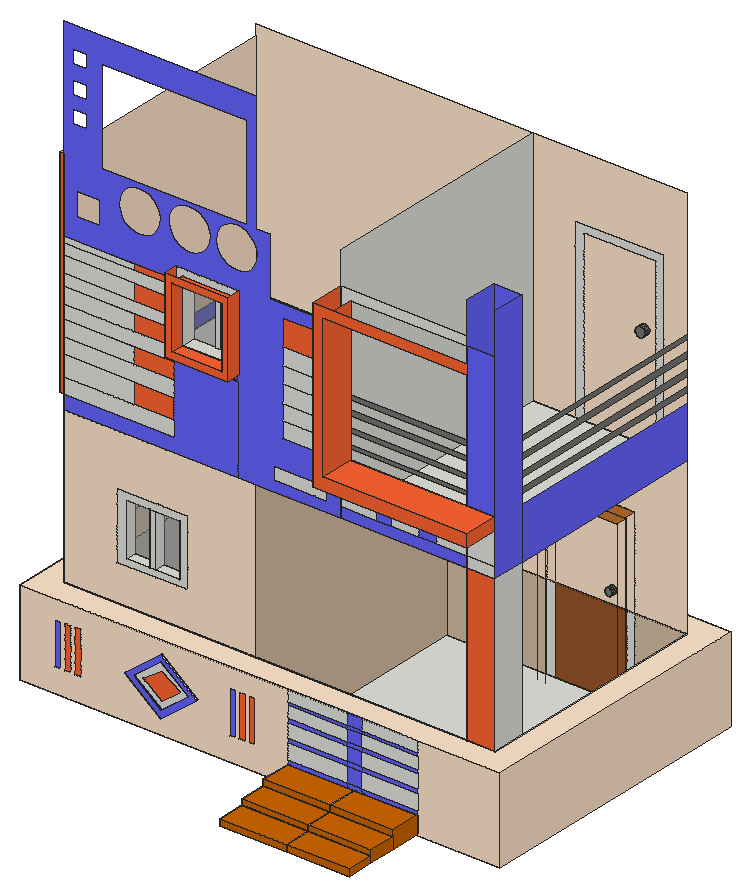
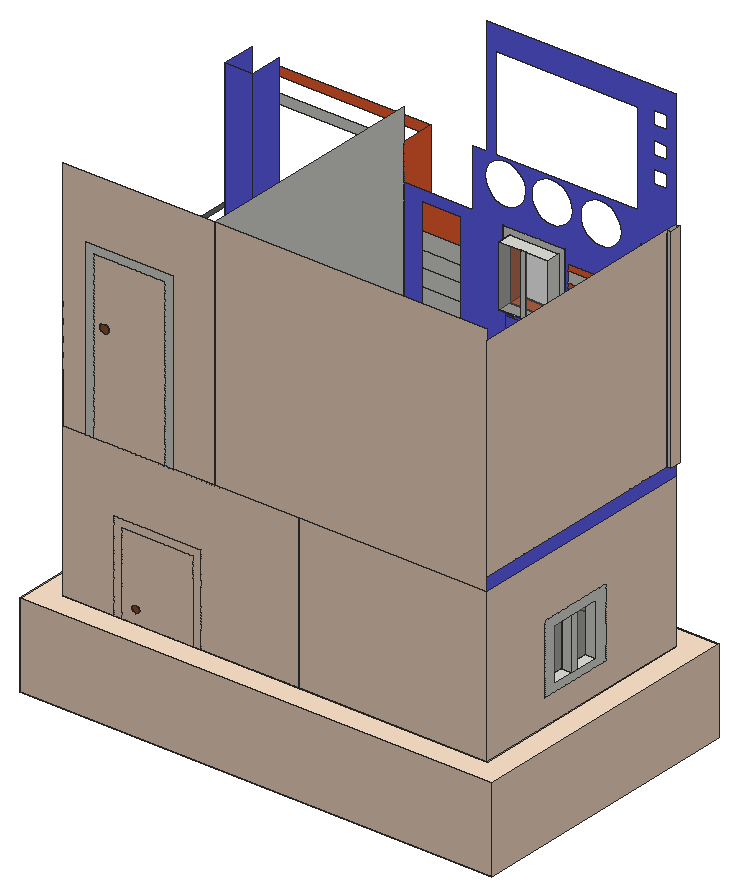
# SketchUp Ruby script. Lengths in inches.
U = 1.inch
M = Sketchup.active_model
def pt(a) = Geom::Point3d.new(a.map { |v| v * U })
def face(e, loops, mat)
  f = e.add_face(loops[0].map { |a| pt(a) })
  loops[1..].each { |l| e.add_face(l.map { |a| pt(a) }).erase! }
  f.material = f.back_material = mat if mat
  f
end
# faces: each face lists its corners as indices into pts; further lists are holes
def faces(e, pts, list, mat = nil) = list.each { |f| face(e, (f[0].is_a?(Array) ? f : [f]).map { |l| l.map { |i| pts[i] } }, mat) }
# xy, xz, yz: faces in a plane at the given z, y or x. An outline is a flat list of corners, or four numbers for a rectangle; further outlines are holes
def ring(l) = l.size == 4 ? [[l[0], l[1]], [l[2], l[1]], [l[2], l[3]], [l[0], l[3]]] : l.each_slice(2).to_a
def flat(e, list, mat, &to3) = list.each { |f| face(e, (f[0].is_a?(Array) ? f : [f]).map { |l| ring(l).map { |u, v| to3.(u, v) } }, mat) }
def xy(e, z, list, mat = nil) = flat(e, list, mat) { |x, y| [x, y, z] }
def xz(e, y, list, mat = nil) = flat(e, list, mat) { |x, z| [x, y, z] }
def yz(e, x, list, mat = nil) = flat(e, list, mat) { |y, z| [x, y, z] }
def lines(e, pts, list) = list.each { |a, b| e.add_line(pt(pts[a]), pt(pts[b])) }
# prism: a flat outline (further loops are holes) pulled along v
def prism(e, loops, v, mat = nil)
  f = face(e, loops, mat); d = Geom::Vector3d.new(v.map { |x| x * U })
  f.pushpull(f.normal.samedirection?(d) ? d.length : -d.length)
end
def box(e, o, s, mat = nil) = prism(e, [[o, [o[0] + s[0], o[1], o[2]], [o[0] + s[0], o[1] + s[1], o[2]], [o[0], o[1] + s[1], o[2]]]], [0, 0, s[2]], mat)
def at(x, y, z, deg = 0) = Geom::Transformation.translation(pt([x, y, z])) * Geom::Transformation.rotation(ORIGIN, Z_AXIS, deg.degrees)
def axes(o, x, y, z) = Geom::Transformation.new([*x, 0, *y, 0, *z, 0, *pt(o).to_a, 1])
def part(name) = M.definitions.add(name)
# library, detail: a bought-in or finely detailed component or shape, given as its bounding box
def library(name, o, s) = part(name).tap { |d| box(d.entities, o, s) }
def detail(e, o, s) = box(e.add_group.entities, o, s)
def put(e, d, t, mat = nil) = e.add_instance(d, t).tap { |i| i.material = mat if mat }
def group(e, t, mat = nil) = e.add_group.tap { |g| g.transformation = t; g.material = mat if mat }.entities
root = M.entities
M.materials.add("[Color B04]").color = [255, 101, 50]
M.materials.add("[Color C01]").color = [255, 229, 204]
M.materials.add("[Color C06]").color = [204, 102, 0]
M.materials.add("[Color I03]").color = [101, 101, 255]
M.materials.add("[Formica Laminate Light]").color = [213, 189, 164]
M.materials.add("[Metal Seamed]").color = [118, 119, 115]
M.materials.add("[Translucent Glass Gray]").color = [128, 128, 128]
M.materials["[Translucent Glass Gray]"].alpha = 0.5
M.materials.add("[Wood Bamboo]").color = [177, 105, 43]
M.materials.add("[Wood Cherry Original]").color = [152, 86, 42]
xy(root,0,[[133.68,0,166.92,13.48],[166.92,0,198.35,13.48],[133.68,13.48,166.92,26.96],[166.92,13.48,198.35,26.96],[133.68,26.96,166.92,42.15],
  [166.92,26.96,198.35,42.15],[[0,42.15,240,186.15],[12,54.15,228,174.15]],[12,54.15,108,174.15],[108,54.15,108,174.15,228,174.15,228,70.82,213.875,70.82,213.875,54.15],[213.875,54.15,228,70.82]])
xy(root,3.25,[[133.68,0,166.92,13.48],[166.92,0,198.35,13.48]],"[Color C06]")
xy(root,6,[[133.68,13.48,166.92,26.96],[166.92,13.48,198.35,26.96]],"[Color C06]")
xy(root,8.9375,[[133.68,26.96,166.92,42.15],[166.92,26.96,198.35,42.15]],"[Color C06]")
xy(root,42.625,[[[0,42.15,240,186.15],[12,54.15,228,174.15]]],"[Color C01]")
xy(root,59.56,[[12,105.09,17.125,117.38],[12,117.38,17.125,120.1],[12,120.1,17.125,131.59]])
xy(root,64.13,[[43.53,54.15,55.36,59.15],[58.01,54.15,70.03,59.15]])
xy(root,84,[[161.79,168.08,197.79,174.15]],"[Wood Bamboo]")
xy(root,86.06,[[12,105.09,17.125,117.38],[12,117.38,17.125,120.1],[12,120.1,17.125,131.59]])
xy(root,88.07,[[157.72,168.08,201.87,174.15]],"[Wood Bamboo]")
xy(root,90.63,[[43.53,54.15,55.36,59.15],[58.01,54.15,70.03,59.15]])
xy(root,120,[[12,54.15,108,174.15],[108,54.15,150.6,174.15],[150.6,54.15,150.6,174.15,228,174.15,228,70.82,213.875,70.82,213.875,54.15],[213.875,54.15,228,70.82]])
xy(root,127.14,[[10.25,54.15,12,59.71]])
xy(root,141.48,[[150.6,36.65,228,54.15]],"[Color B04]")
xy(root,147.71,[[155.5625,36.65,228,54.15]],"[Color B04]")
xy(root,166.23,[[68.34,47.27,99.83,54.15]],"[Color B04]")
xy(root,169.5625,[[71.68,54.15,96.49,61.08]])
xy(root,169.5625,[[71.68,47.27,96.49,54.15]],"[Color B04]")
xy(root,200.625,[[71.68,54.15,96.49,61.08]])
xy(root,200.625,[[71.68,47.27,96.49,54.15]],"[Color B04]")
xz(root,0,[[133.68,0,166.92,3.25],[166.92,0,198.35,3.25]],"[Color C06]")
xz(root,13.48,[[133.68,0,166.92,3.25],[166.92,0,198.35,3.25]])
xz(root,13.48,[[133.68,3.25,166.92,6],[166.92,3.25,198.35,6]],"[Color C06]")
xz(root,26.96,[[133.68,0,166.92,6],[166.92,0,198.35,6]])
xz(root,26.96,[[133.68,6,166.92,8.9375],[166.92,6,198.35,8.9375]],"[Color C06]")
xz(root,36.65,[[150.6,141.48,228,141.48,228,147.71,155.5625,147.71,155.5625,219.21,228,219.21,228,223.92,150.6,223.92]],"[Color B04]")
xz(root,41.21,[[[70.9,7.75,88.86,22.125,70.9,36.5,52.9375,22.125],[70.9,11.17,56.86,22.29,70.9,33.42,84.93,22.29]]],"[Color I03]")
xz(root,42.15,[[133.68,0,163.17,8.9],[163.17,0,166.92,8.9],[166.92,0,170.66,8.9],[170.66,0,198.35,8.9],[198.35,0,199.03,8.9],
  [[70.9,7.75,52.9375,22.125,70.9,36.5,88.86,22.125],[70.9,11.17,84.93,22.29,70.9,33.42,56.86,22.29]],[133.68,8.9,163.17,8.93,163.17,8.9375,133.68,8.9375],[133.68,8.9,163.17,8.93,163.17,8.9],[163.17,8.9,163.17,8.93,166.92,8.9375,166.92,8.9],[166.92,8.9,170.66,8.9375],
  [170.66,8.9,198.35,8.9375],[163.17,8.93,166.92,8.9375,163.17,8.9375],[[70.9,11.17,84.93,22.29,70.9,33.42,56.86,22.29],[70.9,14.9375,61.5,22.29,70.9,28.6875,80.89,22.29]],[133.68,11.17,163.17,18.79],[170.66,11.17,199.03,18.79],
  [133.68,20.98,163.17,27.74],[170.66,20.98,199.03,27.74],[133.68,29.6,163.17,35.43],[170.66,29.6,199.03,35.43],[133.68,37.15,163.17,42.625],
  [170.66,37.15,199.03,42.625]])
xz(root,42.15,[[22.3,11.74,25.43,11.74,25.43,33.17,22.3,33.18],[27.18,11.74,30.3,11.74,30.3,33.17,27.18,33.18],[109.55,11.74,112.68,11.74,112.68,33.17,109.55,33.18],[114.12,11.74,117.24,11.74,117.24,33.17,114.12,33.18],[70.9,14.9375,80.89,22.29,70.9,28.6875,61.5,22.29]],"[Color B04]")
xz(root,42.15,[[[0,0,133.68,42.625],[70.9,7.75,52.9375,22.125,70.9,36.5,88.86,22.125],[17.3,11.74,17.3,33.18,20.43,33.17,20.43,11.74],[22.3,11.74,22.3,33.18,25.43,33.17,25.43,11.74],[27.18,11.74,27.18,33.18,30.3,33.17,30.3,11.74],[104.93,11.74,104.93,33.18,108.05,33.17,108.05,11.74],[109.55,11.74,109.55,33.18,112.68,33.17,112.68,11.74],[114.12,11.74,114.12,33.18,117.24,33.17,117.24,11.74]],[199.03,0,240,42.625]],"[Color C01]")
xz(root,42.15,[[198.35,8.9,199.03,8.9,199.03,11.17,170.66,11.17,170.66,8.9375,198.35,8.9375],[133.68,8.9375,163.17,11.17],[163.17,8.9375,170.66,11.17],[163.17,11.17,170.66,18.79],[17.3,11.74,20.43,11.74,20.43,33.17,17.3,33.18],
  [104.93,11.74,108.05,11.74,108.05,33.17,104.93,33.18],[133.68,18.79,163.17,20.98],[163.17,18.79,170.66,20.98],[170.66,18.79,199.03,20.98],[163.17,20.98,170.66,27.74],
  [133.68,27.74,163.17,29.6],[163.17,27.74,170.66,29.6],[170.66,27.74,199.03,29.6],[163.17,29.6,170.66,35.43],[133.68,35.43,163.17,37.15],
  [163.17,35.43,170.66,37.15],[170.66,35.43,199.03,37.15],[163.17,37.15,170.66,42.625]],"[Color I03]")
xz(root,47.27,[[[68.34,166.23,99.83,203.96],[71.68,169.5625,96.49,200.625]]],"[Color B04]")
xz(root,54.15,[[12,0,108,42.625],[108,0,213.875,42.625],[213.875,0,228,42.625],[[38.72,60.83,74.28,94.14],[43.53,64.13,70.03,90.63]],[55.36,64.13,58.01,90.63],
  [213.875,120,228,125.29],[117.51,125.29,143.21,131.38],[150.6,125.29,168.65,125.29,168.65,129.54,175.53,129.54,175.53,125.29,189.68,125.29,189.68,130.04,198.87,130.04,198.87,125.29,213.875,125.29,213.875,141.48,150.6,141.48],[213.875,125.29,228,141.48],[12,127.14,67.04,134.4375],
  [12,134.4375,47.11,144.6875],[150.6,141.48,150.6,223.92,213.875,223.92,213.875,219.21,155.5625,219.21,155.5625,147.71,213.875,147.71,213.875,141.48],[213.875,141.48,228,147.71],[12,144.6875,67.04,152.5],[121.88,145.48,140.95,153.34],
  [12,152.5,47.11,160.5625],[121.88,153.34,140.95,161.1875],[12,160.5625,67.04,167.25],[121.88,161.1875,140.95,169.8125],[[68.34,166.23,99.83,203.96],[71.68,169.5625,96.49,200.625]],
  [12,167.25,47.11,175.3125],[121.88,169.8125,140.95,178.14],[12,175.3125,67.04,181],[121.88,178.14,140.95,186.65],[12,181,47.11,189.0625],
  [12,189.0625,67.04,194.6875],[12,194.6875,47.11,197.75]])
xz(root,54.15,[[213.875,42.625,228,120],[10.25,127.14,12,234.75],[47.11,134.4375,67.04,144.6875],[47.11,152.5,67.04,160.5625],[69.56,163.46,73.23,166.23],
  [81.22,163.75,85.23,166.23],[93.73,163.8,98.57,166.23],[47.11,167.25,67.04,175.3125],[47.11,181,67.04,189.0625],[121.88,186.65,140.95,199.83],
  [47.11,194.6875,67.04,197.75]],"[Color B04]")
xz(root,54.15,[[[12,42.625,108,120],[38.72,60.83,74.28,94.14]]],"[Color C01]")
xz(root,54.15,[[12,120,99.16,120,99.16,163.08,67.04,163.08,67.04,127.14,12,127.14],[[99.16,120,150.6,120,150.6,205.5625,115.2,205.5625,115.2,234.75,108,234.75,108,294.3125,12,294.3125,12,197.75,67.04,197.75,67.04,163.08,99.16,163.08],[31.45,234.75,103.62,281.875],[69.56,163.46,69.56,166.23,68.34,166.23,68.34,203.96,99.83,203.96,99.83,166.23,98.57,166.23,98.57,163.8,93.73,163.8,93.73,166.23,85.23,166.23,85.23,163.75,81.22,163.75,81.22,166.23,73.23,166.23,73.23,163.46],[121.88,145.48,140.95,199.83],[98.99,212.51,96.28,212.8,93.74,213.79,91.54,215.4,91.24,215.79,89.84,217.53,88.88,219.71,88.74,220.02,88.33,222.71,88.59,225.13,88.62,225.42,89.61,227.96,90.54,229.23,91.22,230.16,93.35,231.87,95.84,232.96,98.53,233.38,101.24,233.08,103.78,232.09,105.98,230.48,107.68,228.36,107.7,228.32,108.78,225.86,109.2,223.17,108.9,220.46,107.91,217.92,106.32,215.75,106.3,215.73,104.18,214.02,101.68,212.92],[50.34,211.64,47.63,211.94,45.09,212.92,42.89,214.53,41.1875,216.66,40.09,219.15,39.68,221.85,39.97,224.55,40.96,227.09,42.57,229.29,44.7,231,47.1875,232.09,49.88,232.51,52.59,232.21,55.13,231.23,57.33,229.61,59.03,227.49,60.13,225,60.55,222.3,60.25,219.59,59.26,217.05,57.65,214.86,55.53,213.15,53.03,212.05],[75.3,212.51,72.59,212.8,70.05,213.79,67.86,215.4,66.15,217.53,65.05,220.02,64.64,222.71,64.93,225.42,65.92,227.96,67.53,230.16,69.66,231.87,72.15,232.96,74.85,233.38,77.55,233.08,80.09,232.09,82.29,230.48,84,228.36,84.01,228.32,85.09,225.86,85.51,223.17,85.21,220.46,84.22,217.92,82.63,215.75,82.61,215.73,80.49,214.02,77.99,212.92],[117.51,125.29,143.21,131.38],[18.78,208.67,30.41,220.29],[16.84,249.64,23.47,256.26],[16.84,262.7,23.47,269.33],[16.84,276.58,23.47,283.2]],[150.6,120,213.875,125.29],[168.65,125.29,175.53,129.54],[189.68,125.29,198.87,130.04],
  [213.875,147.71,228,219.21]],"[Color I03]")
xz(root,54.15,[[155.5625,152.6,213.875,154.59],[155.5625,159.82,213.875,162.13],[155.5625,167.72,213.875,170.01],[155.5625,174.76,213.875,177.06]],"[Metal Seamed]")
xz(root,59.15,[[43.53,64.13,55.36,90.63],[58.01,64.13,70.03,90.63]],"[Translucent Glass Gray]")
xz(root,59.71,[[10.25,127.14,12,234.75]])
xz(root,61.08,[[82.86,169.5625,85.33,200.625]])
xz(root,61.08,[[71.68,169.5625,82.86,200.625],[85.33,169.5625,96.49,200.625]],"[Translucent Glass Gray]")
xz(root,70.82,[[213.875,0,228,120]])
xz(root,70.82,[[213.875,120,228,240]],"[Color I03]")
xz(root,105.09,[[12,59.56,17.125,86.06]])
xz(root,117.38,[[12,59.56,17.125,86.06]])
xz(root,120.1,[[12,59.56,17.125,86.06]])
xz(root,131.59,[[12,59.56,17.125,86.06]])
xz(root,171.21,[[206.59,169.09,207.22,169.13,207.82,169.35,208.35,169.7,208.76,170.1875,209.04,170.76,209.15,171.39,209.11,172.02,208.9,172.62,208.54,173.15,208.05,173.5625,207.48,173.84,206.86,173.95,206.22,173.91,205.62,173.7,205.09,173.34,204.68,172.85,204.4,172.28,204.29,171.65,204.34,171.02,204.55,170.42,204.91,169.89,205.39,169.48,205.96,169.2]],"[Metal Seamed]")
xz(root,171.52,[[190.81,47.53,191.29,47.6,191.74,47.78,192.13,48.08,192.43,48.47,192.62,48.92,192.68,49.41,192.62,49.89,192.43,50.34,192.13,50.73,191.74,51.03,191.29,51.22,190.81,51.28,190.32,51.22,189.87,51.03,189.48,50.73,189.18,50.34,188.99,49.89,188.93,49.41,188.99,48.92,189.18,48.47,189.48,48.08,189.87,47.78,190.32,47.6]],"[Metal Seamed]")
xz(root,174.15,[[12,0,108,42.625],[157.72,0,161.79,42.625],[197.79,0,201.87,42.625],[171.88,120,171.88,208.17,216.22,208.17,216.22,120,212.05,120,212.05,204,176.05,204,176.05,120]])
xz(root,174.15,[[12,42.625,108,120],[108,42.625,108,120,228,120,228,42.625,201.87,42.625,201.87,88.07,157.72,88.07,157.72,42.625],[157.72,42.625,157.72,88.07,201.87,88.07,201.87,42.625,197.79,42.625,197.79,84,161.79,84,161.79,42.625],[[161.79,42.625,197.79,84],[190.81,47.53,191.29,47.6,191.74,47.78,192.13,48.08,192.43,48.47,192.62,48.92,192.68,49.41,192.62,49.89,192.43,50.34,192.13,50.73,191.74,51.03,191.29,51.22,190.81,51.28,190.32,51.22,189.87,51.03,189.48,50.73,189.18,50.34,188.99,49.89,188.93,49.41,188.99,48.92,189.18,48.47,189.48,48.08,189.87,47.78,190.32,47.6]],[12,120,150.6,240],
  [150.6,120,150.6,240,228,240,228,120,216.22,120,216.22,208.17,171.88,208.17,171.88,120],[[176.05,120,212.05,204],[206.59,169.09,207.22,169.13,207.82,169.35,208.35,169.7,208.76,170.1875,209.04,170.76,209.15,171.39,209.11,172.02,208.9,172.62,208.54,173.15,208.05,173.5625,207.48,173.84,206.86,173.95,206.22,173.91,205.62,173.7,205.09,173.34,204.68,172.85,204.4,172.28,204.29,171.65,204.34,171.02,204.55,170.42,204.91,169.89,205.39,169.48,205.96,169.2]]],"[Color C01]")
xz(root,174.15,[[108,0,157.72,42.625],[201.87,0,228,42.625]],"[Formica Laminate Light]")
xz(root,174.15,[[161.79,0,197.79,42.625],[190.81,47.53,190.32,47.6,189.87,47.78,189.48,48.08,189.18,48.47,188.99,48.92,188.93,49.41,188.99,49.89,189.18,50.34,189.48,50.73,189.87,51.03,190.32,51.22,190.81,51.28,191.29,51.22,191.74,51.03,192.13,50.73,192.43,50.34,192.62,49.89,192.68,49.41,192.62,48.92,192.43,48.47,192.13,48.08,191.74,47.78,191.29,47.6],[206.59,169.09,205.96,169.2,205.39,169.48,204.91,169.89,204.55,170.42,204.34,171.02,204.29,171.65,204.4,172.28,204.68,172.85,205.09,173.34,205.62,173.7,206.22,173.91,206.86,173.95,207.48,173.84,208.05,173.5625,208.54,173.15,208.9,172.62,209.11,172.02,209.15,171.39,209.04,170.76,208.76,170.1875,208.35,169.7,207.82,169.35,207.22,169.13]],"[Wood Cherry Original]")
xz(root,186.15,[[0,0,240,42.625]],"[Color C01]")
yz(root,0,[[42.15,0,186.15,42.625]],"[Color C01]")
yz(root,10.25,[[54.15,127.14,59.71,234.75]],"[Color C01]")
yz(root,12,[[54.15,0,174.15,42.625],[[98.99,55.92,137.37,91.04],[105.09,59.56,131.59,86.06]],[117.38,59.56,120.1,86.06],[54.15,127.14,59.71,234.75]])
yz(root,12,[[[54.15,42.625,174.15,120],[98.99,55.92,137.37,91.04]],[59.71,127.14,174.15,234.75]],"[Color C01]")
yz(root,12,[[54.15,120,174.15,127.14]],"[Color I03]")
yz(root,17.125,[[117.38,59.56,120.1,86.06]])
yz(root,17.125,[[105.09,59.56,117.38,86.06],[120.1,59.56,131.59,86.06]],"[Translucent Glass Gray]")
yz(root,43.53,[[54.15,64.13,59.15,90.63]])
yz(root,55.36,[[54.15,64.13,59.15,90.63]])
yz(root,58.01,[[54.15,64.13,59.15,90.63]])
yz(root,68.34,[[47.27,166.23,54.15,203.96]],"[Color B04]")
yz(root,70.03,[[54.15,64.13,59.15,90.63]])
yz(root,71.68,[[54.15,169.5625,61.08,200.625]])
yz(root,71.68,[[47.27,169.5625,54.15,200.625]],"[Color B04]")
yz(root,96.49,[[54.15,169.5625,61.08,200.625]])
yz(root,96.49,[[47.27,169.5625,54.15,200.625]],"[Color B04]")
yz(root,99.83,[[47.27,166.23,54.15,203.96]],"[Color B04]")
yz(root,108,[[54.15,0,174.15,120]],"[Formica Laminate Light]")
yz(root,133.68,[[0,0,13.48,3.25],[13.48,0,26.96,6],[26.96,0,42.15,8.9375]],"[Color C06]")
yz(root,150.6,[[54.15,120,174.15,240]])
yz(root,150.6,[[36.65,141.48,54.15,223.92]],"[Color B04]")
yz(root,155.5625,[[36.65,147.71,54.15,219.21]],"[Color B04]")
yz(root,166.92,[[0,0,13.48,3.25],[13.48,0,26.96,0,26.96,6,20.38,6,13.48,5.07],[26.96,0,42.15,0,42.15,8.9375,26.96,6.89],[13.48,5.07,13.48,6,20.38,6],[26.96,6.89,42.15,8.9375,26.96,8.9375]])
yz(root,198.35,[[0,0,13.48,3.25],[13.48,0,26.96,6],[26.96,0,42.15,8.9375]],"[Color C06]")
yz(root,213.875,[[54.15,0,70.82,120]])
yz(root,213.875,[[54.15,120,70.82,240]],"[Color I03]")
yz(root,228,[[54.15,0,70.82,42.625],[70.82,0,174.15,42.625],[54.15,42.625,70.82,120]])
yz(root,228,[[36.65,141.48,54.15,147.71]],"[Color B04]")
yz(root,228,[[54.15,120,70.82,240],[70.82,120,174.15,145.8125]],"[Color I03]")
yz(root,228,[[70.82,150.81,174.15,153.29],[70.82,157.79,174.15,160.68],[70.82,165.84,174.15,168.79],[70.82,174.27,174.15,176.66]],"[Metal Seamed]")
yz(root,240,[[42.15,0,186.15,42.625]],"[Color C01]")
p = [[52.9375,42.15,22.125],[70.9,42.15,7.75],[70.9,41.21,7.75],[52.9375,41.21,22.125],[88.86,42.15,22.125],[88.86,41.21,22.125],
  [70.9,42.15,11.17],[56.86,42.15,22.29],[56.86,41.21,22.29],[70.9,41.21,11.17],[84.93,42.15,22.29],[84.93,41.21,22.29],
  [70.9,42.15,36.5],[70.9,41.21,36.5],[70.9,42.15,33.42],[70.9,41.21,33.42],[190.32,174.15,47.6],[190.81,174.15,47.53],
  [190.81,171.52,47.53],[190.32,171.52,47.6],[191.29,174.15,47.6],[191.29,171.52,47.6],[189.87,174.15,47.78],[189.87,171.52,47.78],
  [191.74,174.15,47.78],[191.74,171.52,47.78],[189.48,174.15,48.08],[189.48,171.52,48.08],[192.13,174.15,48.08],[192.13,171.52,48.08],
  [189.18,174.15,48.47],[189.18,171.52,48.47],[192.43,174.15,48.47],[192.43,171.52,48.47],[188.99,174.15,48.92],[188.99,171.52,48.92],
  [192.62,174.15,48.92],[192.62,171.52,48.92],[188.93,174.15,49.41],[188.93,171.52,49.41],[192.68,174.15,49.41],[192.68,171.52,49.41],
  [188.99,174.15,49.89],[188.99,171.52,49.89],[192.62,174.15,49.89],[192.62,171.52,49.89],[189.18,174.15,50.34],[189.18,171.52,50.34],
  [192.43,174.15,50.34],[192.43,171.52,50.34],[189.48,174.15,50.73],[189.48,171.52,50.73],[192.13,174.15,50.73],[192.13,171.52,50.73],
  [189.87,174.15,51.03],[189.87,171.52,51.03],[191.74,174.15,51.03],[191.74,171.52,51.03],[190.32,174.15,51.22],[190.32,171.52,51.22],
  [191.29,174.15,51.22],[191.29,171.52,51.22],[190.81,174.15,51.28],[190.81,171.52,51.28],[205.96,174.15,169.2],[206.59,174.15,169.09],
  [206.59,171.21,169.09],[205.96,171.21,169.2],[207.22,174.15,169.13],[207.22,171.21,169.13],[207.82,174.15,169.35],[207.82,171.21,169.35],
  [205.39,174.15,169.48],[205.39,171.21,169.48],[208.35,174.15,169.7],[208.35,171.21,169.7],[204.91,174.15,169.89],[204.91,171.21,169.89],
  [208.76,174.15,170.1875],[208.76,171.21,170.1875],[204.55,174.15,170.42],[204.55,171.21,170.42],[209.04,174.15,170.76],[209.04,171.21,170.76],
  [204.34,174.15,171.02],[204.34,171.21,171.02],[209.15,174.15,171.39],[209.15,171.21,171.39],[204.29,174.15,171.65],[204.29,171.21,171.65],
  [209.11,174.15,172.02],[209.11,171.21,172.02],[204.4,174.15,172.28],[204.4,171.21,172.28],[208.9,174.15,172.62],[208.9,171.21,172.62],
  [204.68,174.15,172.85],[204.68,171.21,172.85],[208.54,174.15,173.15],[208.54,171.21,173.15],[205.09,174.15,173.34],[205.09,171.21,173.34],
  [208.05,174.15,173.5625],[208.05,171.21,173.5625],[205.62,174.15,173.7],[205.62,171.21,173.7],[207.48,174.15,173.84],[207.48,171.21,173.84],
  [206.22,174.15,173.91],[206.22,171.21,173.91],[206.86,174.15,173.95],[206.86,171.21,173.95],[157.72,168.08,88.07],[157.72,168.08,0],
  [201.87,168.08,0],[201.87,168.08,88.07],[197.79,168.08,0],[197.79,168.08,84],[161.79,168.08,84],[161.79,168.08,0]]
faces(root,p,[[0,1,2,3],[1,4,5,2],[6,7,8,9],[10,6,9,11],[12,0,3,13],[4,12,13,5],[7,14,15,8],[14,10,11,15]])
faces(root,p,[[16,17,18,19],[17,20,21,18],[22,16,19,23],[20,24,25,21],[26,22,23,27],[24,28,29,25],[30,26,27,31],[28,32,33,29],
  [34,30,31,35],[32,36,37,33],[38,34,35,39],[36,40,41,37],[42,38,39,43],[40,44,45,41],[46,42,43,47],[44,48,49,45],
  [50,46,47,51],[48,52,53,49],[54,50,51,55],[52,56,57,53],[58,54,55,59],[56,60,61,57],[62,58,59,63],[60,62,63,61],
  [64,65,66,67],[65,68,69,66],[68,70,71,69],[72,64,67,73],[70,74,75,71],[76,72,73,77],[74,78,79,75],[80,76,77,81],
  [78,82,83,79],[84,80,81,85],[82,86,87,83],[88,84,85,89],[86,90,91,87],[92,88,89,93],[90,94,95,91],[96,92,93,97],
  [94,98,99,95],[100,96,97,101],[98,102,103,99],[104,100,101,105],[102,106,107,103],[108,104,105,109],[106,110,111,107],[110,108,109,111]],"[Metal Seamed]")
lines(root,p,[[112,113],[114,115],[116,117],[118,119]])
